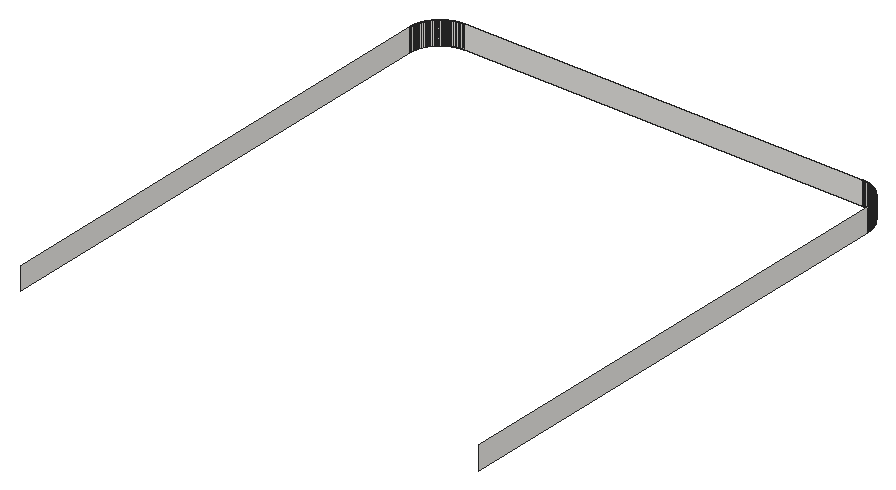
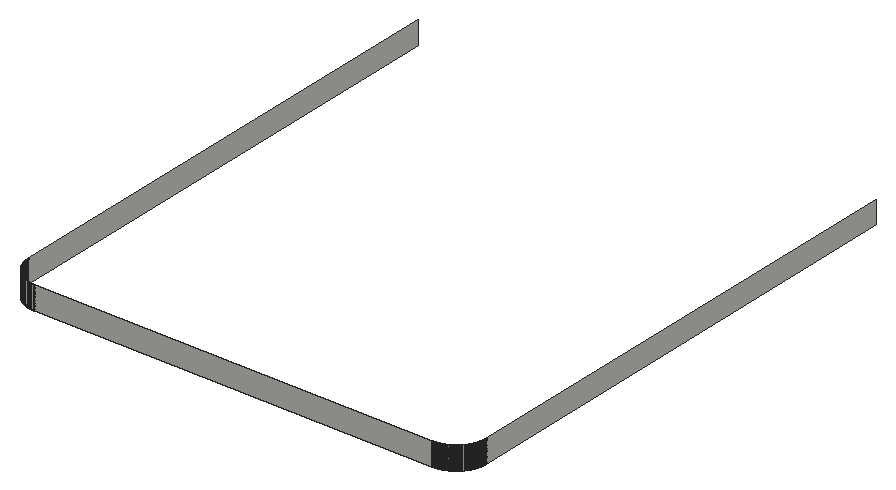
# SketchUp Ruby script. Lengths in inches.
U = 1.inch
M = Sketchup.active_model
def pt(a) = Geom::Point3d.new(a.map { |v| v * U })
def face(e, loops, mat)
  f = e.add_face(loops[0].map { |a| pt(a) })
  loops[1..].each { |l| e.add_face(l.map { |a| pt(a) }).erase! }
  f.material = f.back_material = mat if mat
  f
end
# faces: each face lists its corners as indices into pts; further lists are holes
def faces(e, pts, list, mat = nil) = list.each { |f| face(e, (f[0].is_a?(Array) ? f : [f]).map { |l| l.map { |i| pts[i] } }, mat) }
# xy, xz, yz: faces in a plane at the given z, y or x. An outline is a flat list of corners, or four numbers for a rectangle; further outlines are holes
def ring(l) = l.size == 4 ? [[l[0], l[1]], [l[2], l[1]], [l[2], l[3]], [l[0], l[3]]] : l.each_slice(2).to_a
def flat(e, list, mat, &to3) = list.each { |f| face(e, (f[0].is_a?(Array) ? f : [f]).map { |l| ring(l).map { |u, v| to3.(u, v) } }, mat) }
def xy(e, z, list, mat = nil) = flat(e, list, mat) { |x, y| [x, y, z] }
def xz(e, y, list, mat = nil) = flat(e, list, mat) { |x, z| [x, y, z] }
def yz(e, x, list, mat = nil) = flat(e, list, mat) { |y, z| [x, y, z] }
def lines(e, pts, list) = list.each { |a, b| e.add_line(pt(pts[a]), pt(pts[b])) }
# prism: a flat outline (further loops are holes) pulled along v
def prism(e, loops, v, mat = nil)
  f = face(e, loops, mat); d = Geom::Vector3d.new(v.map { |x| x * U })
  f.pushpull(f.normal.samedirection?(d) ? d.length : -d.length)
end
def box(e, o, s, mat = nil) = prism(e, [[o, [o[0] + s[0], o[1], o[2]], [o[0] + s[0], o[1] + s[1], o[2]], [o[0], o[1] + s[1], o[2]]]], [0, 0, s[2]], mat)
def at(x, y, z, deg = 0) = Geom::Transformation.translation(pt([x, y, z])) * Geom::Transformation.rotation(ORIGIN, Z_AXIS, deg.degrees)
def axes(o, x, y, z) = Geom::Transformation.new([*x, 0, *y, 0, *z, 0, *pt(o).to_a, 1])
def part(name) = M.definitions.add(name)
# library, detail: a bought-in or finely detailed component or shape, given as its bounding box
def library(name, o, s) = part(name).tap { |d| box(d.entities, o, s) }
def detail(e, o, s) = box(e.add_group.entities, o, s)
def put(e, d, t, mat = nil) = e.add_instance(d, t).tap { |i| i.material = mat if mat }
def group(e, t, mat = nil) = e.add_group.tap { |g| g.transformation = t; g.material = mat if mat }.entities
root = M.entities
M.materials.add("[Formica Graystone]").color = [224, 223, 219]
xz(root,444,[[17.6875,383.82,17.84,392.82],[17.84,383.82,18,392.82],[18,383.82,174,392.82],[174,383.82,174.16,392.82],[174.16,383.82,174.3125,392.82]],"[Formica Graystone]")
yz(root,6,[[241,383.82,432,392.82],[432,383.82,432.16,392.82],[432.16,383.82,432.3125,392.82]],"[Formica Graystone]")
yz(root,186,[[241,383.82,432,392.82],[432,383.82,432.16,392.82],[432.16,383.82,432.3125,392.82]],"[Formica Graystone]")
p = [[6.01,432.47,383.82],[6,432.3125,383.82],[6,432.3125,392.82],[6.01,432.47,392.82],[186,432.3125,383.82],[185.99,432.47,383.82],
  [185.99,432.47,392.82],[186,432.3125,392.82],[6.02,432.63,383.82],[6.02,432.63,392.82],[185.98,432.63,383.82],[185.98,432.63,392.82],
  [6.03,432.78,383.82],[6.03,432.78,392.82],[185.97,432.78,383.82],[185.97,432.78,392.82],[6.04,432.94,383.82],[6.04,432.94,392.82],
  [185.96,432.94,383.82],[185.96,432.94,392.82],[6.05,433.1,383.82],[6.05,433.1,392.82],[185.95,433.1,383.82],[185.95,433.1,392.82],
  [6.07,433.25,383.82],[6.07,433.25,392.82],[185.93,433.25,383.82],[185.93,433.25,392.82],[6.08,433.41,383.82],[6.08,433.41,392.82],
  [185.92,433.41,383.82],[185.92,433.41,392.82],[6.1,433.57,383.82],[6.1,433.57,392.82],[185.9,433.57,383.82],[185.9,433.57,392.82],
  [6.125,433.72,383.82],[6.125,433.72,392.82],[185.875,433.72,383.82],[185.875,433.72,392.82],[6.15,433.88,383.82],[6.15,433.88,392.82],
  [185.85,433.88,383.82],[185.85,433.88,392.82],[6.17,434.03,383.82],[6.17,434.03,392.82],[185.83,434.03,383.82],[185.83,434.03,392.82],
  [6.2,434.1875,383.82],[6.2,434.1875,392.82],[185.8,434.1875,383.82],[185.8,434.1875,392.82],[6.23,434.34,383.82],[6.23,434.34,392.82],
  [185.77,434.34,383.82],[185.77,434.34,392.82],[6.26,434.49,383.82],[6.26,434.49,392.82],[185.74,434.49,383.82],[185.74,434.49,392.82],
  [6.3,434.65,383.82],[6.3,434.65,392.82],[185.7,434.65,383.82],[185.7,434.65,392.82],[6.33,434.8,383.82],[6.33,434.8,392.82],
  [185.67,434.8,383.82],[185.67,434.8,392.82],[6.37,434.95,383.82],[6.37,434.95,392.82],[185.63,434.95,383.82],[185.63,434.95,392.82],
  [6.41,435.11,383.82],[6.41,435.11,392.82],[185.59,435.11,383.82],[185.59,435.11,392.82],[6.45,435.26,383.82],[6.45,435.26,392.82],
  [185.55,435.26,383.82],[185.55,435.26,392.82],[6.49,435.41,383.82],[6.49,435.41,392.82],[185.51,435.41,383.82],[185.51,435.41,392.82],
  [6.54,435.56,383.82],[6.54,435.56,392.82],[185.46,435.56,383.82],[185.46,435.56,392.82],[6.59,435.71,383.82],[6.59,435.71,392.82],
  [185.41,435.71,383.82],[185.41,435.71,392.82],[6.64,435.86,383.82],[6.64,435.86,392.82],[185.36,435.86,383.82],[185.36,435.86,392.82],
  [6.6875,436.01,383.82],[6.6875,436.01,392.82],[185.3125,436.01,383.82],[185.3125,436.01,392.82],[6.74,436.15,383.82],[6.74,436.15,392.82],
  [185.26,436.15,383.82],[185.26,436.15,392.82],[6.8,436.3,383.82],[6.8,436.3,392.82],[185.2,436.3,383.82],[185.2,436.3,392.82],
  [6.85,436.45,383.82],[6.85,436.45,392.82],[185.15,436.45,383.82],[185.15,436.45,392.82],[6.91,436.59,383.82],[6.91,436.59,392.82],
  [185.09,436.59,383.82],[185.09,436.59,392.82],[6.97,436.74,383.82],[6.97,436.74,392.82],[185.03,436.74,383.82],[185.03,436.74,392.82],
  [7.04,436.88,383.82],[7.04,436.88,392.82],[184.96,436.88,383.82],[184.96,436.88,392.82],[7.1,437.02,383.82],[7.1,437.02,392.82],
  [184.9,437.02,383.82],[184.9,437.02,392.82],[7.17,437.17,383.82],[7.17,437.17,392.82],[184.83,437.17,383.82],[184.83,437.17,392.82],
  [7.24,437.31,383.82],[7.24,437.31,392.82],[184.76,437.31,383.82],[184.76,437.31,392.82],[7.31,437.45,383.82],[7.31,437.45,392.82],
  [184.69,437.45,383.82],[184.69,437.45,392.82],[7.38,437.59,383.82],[7.38,437.59,392.82],[184.62,437.59,383.82],[184.62,437.59,392.82],
  [7.45,437.73,383.82],[7.45,437.73,392.82],[184.55,437.73,383.82],[184.55,437.73,392.82],[7.53,437.86,383.82],[7.53,437.86,392.82],
  [184.47,437.86,383.82],[184.47,437.86,392.82],[7.61,438,383.82],[7.61,438,392.82],[184.39,438,383.82],[184.39,438,392.82],
  [7.6875,438.14,383.82],[7.6875,438.14,392.82],[184.3125,438.14,383.82],[184.3125,438.14,392.82],[7.77,438.27,383.82],[7.77,438.27,392.82],
  [184.23,438.27,383.82],[184.23,438.27,392.82],[7.85,438.4,383.82],[7.85,438.4,392.82],[184.15,438.4,383.82],[184.15,438.4,392.82],
  [7.9375,438.54,383.82],[7.9375,438.54,392.82],[184.0625,438.54,383.82],[184.0625,438.54,392.82],[8.02,438.67,383.82],[8.02,438.67,392.82],
  [183.98,438.67,383.82],[183.98,438.67,392.82],[8.11,438.8,383.82],[8.11,438.8,392.82],[183.89,438.8,383.82],[183.89,438.8,392.82],
  [8.2,438.93,383.82],[8.2,438.93,392.82],[183.8,438.93,383.82],[183.8,438.93,392.82],[8.29,439.05,383.82],[8.29,439.05,392.82],
  [183.71,439.05,383.82],[183.71,439.05,392.82],[8.38,439.18,383.82],[8.38,439.18,392.82],[183.62,439.18,383.82],[183.62,439.18,392.82],
  [8.48,439.31,383.82],[8.48,439.31,392.82],[183.52,439.31,383.82],[183.52,439.31,392.82],[8.58,439.43,383.82],[8.58,439.43,392.82],
  [183.42,439.43,383.82],[183.42,439.43,392.82],[8.67,439.55,383.82],[8.67,439.55,392.82],[183.33,439.55,383.82],[183.33,439.55,392.82],
  [8.77,439.67,383.82],[8.77,439.67,392.82],[183.23,439.67,383.82],[183.23,439.67,392.82],[8.875,439.79,383.82],[8.875,439.79,392.82],
  [183.125,439.79,383.82],[183.125,439.79,392.82],[8.98,439.91,383.82],[8.98,439.91,392.82],[183.02,439.91,383.82],[183.02,439.91,392.82],
  [9.08,440.03,383.82],[9.08,440.03,392.82],[182.92,440.03,383.82],[182.92,440.03,392.82],[9.1875,440.15,383.82],[9.1875,440.15,392.82],
  [182.8125,440.15,383.82],[182.8125,440.15,392.82],[9.3,440.26,383.82],[9.3,440.26,392.82],[182.7,440.26,383.82],[182.7,440.26,392.82],
  [9.4,440.375,383.82],[9.4,440.375,392.82],[182.6,440.375,383.82],[182.6,440.375,392.82],[9.51,440.49,383.82],[9.51,440.49,392.82],
  [182.49,440.49,383.82],[182.49,440.49,392.82],[9.625,440.6,383.82],[9.625,440.6,392.82],[182.375,440.6,383.82],[182.375,440.6,392.82],
  [9.74,440.7,383.82],[9.74,440.7,392.82],[182.26,440.7,383.82],[182.26,440.7,392.82],[9.85,440.8125,383.82],[9.85,440.8125,392.82],
  [182.15,440.8125,383.82],[182.15,440.8125,392.82],[9.97,440.92,383.82],[9.97,440.92,392.82],[182.03,440.92,383.82],[182.03,440.92,392.82],
  [10.09,441.02,383.82],[10.09,441.02,392.82],[181.91,441.02,383.82],[181.91,441.02,392.82],[10.21,441.125,383.82],[10.21,441.125,392.82],
  [181.79,441.125,383.82],[181.79,441.125,392.82],[10.33,441.23,383.82],[10.33,441.23,392.82],[181.67,441.23,383.82],[181.67,441.23,392.82],
  [10.45,441.33,383.82],[10.45,441.33,392.82],[181.55,441.33,383.82],[181.55,441.33,392.82],[10.57,441.42,383.82],[10.57,441.42,392.82],
  [181.43,441.42,383.82],[181.43,441.42,392.82],[10.69,441.52,383.82],[10.69,441.52,392.82],[181.31,441.52,383.82],[181.31,441.52,392.82],
  [10.82,441.62,383.82],[10.82,441.62,392.82],[181.18,441.62,383.82],[181.18,441.62,392.82],[10.95,441.71,383.82],[10.95,441.71,392.82],
  [181.05,441.71,383.82],[181.05,441.71,392.82],[11.07,441.8,383.82],[11.07,441.8,392.82],[180.93,441.8,383.82],[180.93,441.8,392.82],
  [11.2,441.89,383.82],[11.2,441.89,392.82],[180.8,441.89,383.82],[180.8,441.89,392.82],[11.33,441.98,383.82],[11.33,441.98,392.82],
  [180.67,441.98,383.82],[180.67,441.98,392.82],[11.46,442.0625,383.82],[11.46,442.0625,392.82],[180.54,442.0625,383.82],[180.54,442.0625,392.82],
  [11.6,442.15,383.82],[11.6,442.15,392.82],[11.73,442.23,383.82],[11.73,442.23,392.82],[180.4,442.15,383.82],[180.27,442.23,383.82],
  [180.27,442.23,392.82],[180.4,442.15,392.82],[11.86,442.3125,383.82],[11.86,442.3125,392.82],[180.14,442.3125,383.82],[180.14,442.3125,392.82],
  [12,442.39,383.82],[12,442.39,392.82],[180,442.39,383.82],[180,442.39,392.82],[12.14,442.47,383.82],[12.14,442.47,392.82],
  [179.86,442.47,383.82],[179.86,442.47,392.82],[12.27,442.55,383.82],[12.27,442.55,392.82],[12.41,442.62,383.82],[12.41,442.62,392.82],
  [179.73,442.55,383.82],[179.59,442.62,383.82],[179.59,442.62,392.82],[179.73,442.55,392.82],[12.55,442.69,383.82],[12.55,442.69,392.82],
  [179.45,442.69,383.82],[179.45,442.69,392.82],[12.69,442.76,383.82],[12.69,442.76,392.82],[179.31,442.76,383.82],[179.31,442.76,392.82],
  [12.83,442.83,383.82],[12.83,442.83,392.82],[12.98,442.9,383.82],[12.98,442.9,392.82],[179.17,442.83,383.82],[179.02,442.9,383.82],
  [179.02,442.9,392.82],[179.17,442.83,392.82],[13.12,442.96,383.82],[13.12,442.96,392.82],[178.88,442.96,383.82],[178.88,442.96,392.82],
  [13.26,443.03,383.82],[13.26,443.03,392.82],[13.41,443.09,383.82],[13.41,443.09,392.82],[178.74,443.03,383.82],[178.59,443.09,383.82],
  [178.59,443.09,392.82],[178.74,443.03,392.82],[13.55,443.15,383.82],[13.55,443.15,392.82],[13.7,443.2,383.82],[13.7,443.2,392.82],
  [178.45,443.15,383.82],[178.3,443.2,383.82],[178.3,443.2,392.82],[178.45,443.15,392.82],[13.85,443.26,383.82],[13.85,443.26,392.82],
  [178.15,443.26,383.82],[178.15,443.26,392.82],[13.99,443.3125,383.82],[13.99,443.3125,392.82],[14.14,443.36,383.82],[14.14,443.36,392.82],
  [178.01,443.3125,383.82],[177.86,443.36,383.82],[177.86,443.36,392.82],[178.01,443.3125,392.82],[14.29,443.41,383.82],[14.29,443.41,392.82],
  [14.44,443.46,383.82],[14.44,443.46,392.82],[177.71,443.41,383.82],[177.56,443.46,383.82],[177.56,443.46,392.82],[177.71,443.41,392.82],
  [14.59,443.51,383.82],[14.59,443.51,392.82],[14.74,443.55,383.82],[14.74,443.55,392.82],[14.89,443.59,383.82],[14.89,443.59,392.82],
  [177.26,443.55,383.82],[177.11,443.59,383.82],[177.11,443.59,392.82],[177.26,443.55,392.82],[177.41,443.51,383.82],[177.41,443.51,392.82],
  [15.05,443.63,383.82],[15.05,443.63,392.82],[15.2,443.67,383.82],[15.2,443.67,392.82],[176.95,443.63,383.82],[176.8,443.67,383.82],
  [176.8,443.67,392.82],[176.95,443.63,392.82],[15.35,443.7,383.82],[15.35,443.7,392.82],[15.51,443.74,383.82],[15.51,443.74,392.82],
  [15.66,443.77,383.82],[15.66,443.77,392.82],[176.49,443.74,383.82],[176.34,443.77,383.82],[176.34,443.77,392.82],[176.49,443.74,392.82],
  [176.65,443.7,383.82],[176.65,443.7,392.82],[15.8125,443.8,383.82],[15.8125,443.8,392.82],[15.97,443.83,383.82],[15.97,443.83,392.82],
  [16.12,443.85,383.82],[16.12,443.85,392.82],[176.03,443.83,383.82],[175.88,443.85,383.82],[175.88,443.85,392.82],[176.03,443.83,392.82],
  [176.1875,443.8,383.82],[176.1875,443.8,392.82],[16.28,443.875,383.82],[16.28,443.875,392.82],[16.43,443.9,383.82],[16.43,443.9,392.82],
  [16.59,443.92,383.82],[16.59,443.92,392.82],[16.75,443.93,383.82],[16.75,443.93,392.82],[16.9,443.95,383.82],[16.9,443.95,392.82],
  [17.06,443.96,383.82],[17.06,443.96,392.82],[175.1,443.95,383.82],[174.94,443.96,383.82],[174.94,443.96,392.82],[175.1,443.95,392.82],
  [175.25,443.93,383.82],[175.25,443.93,392.82],[175.41,443.92,383.82],[175.41,443.92,392.82],[175.57,443.9,383.82],[175.57,443.9,392.82],
  [175.72,443.875,383.82],[175.72,443.875,392.82],[17.22,443.97,383.82],[17.22,443.97,392.82],[17.37,443.98,383.82],[17.37,443.98,392.82],
  [17.53,443.99,383.82],[17.53,443.99,392.82],[17.6875,444,383.82],[17.6875,444,392.82],[174.47,443.99,383.82],[174.3125,444,383.82],
  [174.3125,444,392.82],[174.47,443.99,392.82],[174.63,443.98,383.82],[174.63,443.98,392.82],[174.78,443.97,383.82],[174.78,443.97,392.82]]
faces(root,p,[[0,1,2,3],[4,5,6,7],[8,0,3,9],[5,10,11,6],[12,8,9,13],[10,14,15,11],[16,12,13,17],[14,18,19,15],
  [20,16,17,21],[18,22,23,19],[24,20,21,25],[22,26,27,23],[28,24,25,29],[26,30,31,27],[32,28,29,33],[30,34,35,31],
  [36,32,33,37],[34,38,39,35],[40,36,37,41],[38,42,43,39],[44,40,41,45],[42,46,47,43],[48,44,45,49],[46,50,51,47],
  [52,48,49,53],[50,54,55,51],[56,52,53,57],[54,58,59,55],[60,56,57,61],[58,62,63,59],[64,60,61,65],[62,66,67,63],
  [68,64,65,69],[66,70,71,67],[72,68,69,73],[70,74,75,71],[76,72,73,77],[74,78,79,75],[80,76,77,81],[78,82,83,79],
  [84,80,81,85],[82,86,87,83],[88,84,85,89],[86,90,91,87],[92,88,89,93],[90,94,95,91],[96,92,93,97],[94,98,99,95],
  [100,96,97,101],[98,102,103,99],[104,100,101,105],[102,106,107,103],[108,104,105,109],[106,110,111,107],[112,108,109,113],[110,114,115,111],
  [116,112,113,117],[114,118,119,115],[120,116,117,121],[118,122,123,119],[124,120,121,125],[122,126,127,123],[128,124,125,129],[126,130,131,127],
  [132,128,129,133],[130,134,135,131],[136,132,133,137],[134,138,139,135],[140,136,137,141],[138,142,143,139],[144,140,141,145],[142,146,147,143],
  [148,144,145,149],[146,150,151,147],[152,148,149,153],[150,154,155,151],[156,152,153,157],[154,158,159,155],[160,156,157,161],[158,162,163,159],
  [164,160,161,165],[162,166,167,163],[168,164,165,169],[166,170,171,167],[172,168,169,173],[170,174,175,171],[176,172,173,177],[174,178,179,175],
  [180,176,177,181],[178,182,183,179],[184,180,181,185],[182,186,187,183],[188,184,185,189],[186,190,191,187],[192,188,189,193],[190,194,195,191],
  [196,192,193,197],[194,198,199,195],[200,196,197,201],[198,202,203,199],[204,200,201,205],[202,206,207,203],[208,204,205,209],[206,210,211,207],
  [212,208,209,213],[210,214,215,211],[216,212,213,217],[214,218,219,215],[220,216,217,221],[218,222,223,219],[224,220,221,225],[222,226,227,223],
  [228,224,225,229],[226,230,231,227],[232,228,229,233],[230,234,235,231],[236,232,233,237],[234,238,239,235],[240,236,237,241],[238,242,243,239],
  [244,240,241,245],[242,246,247,243],[248,244,245,249],[246,250,251,247],[252,248,249,253],[250,254,255,251],[256,252,253,257],[254,258,259,255],
  [260,256,257,261],[258,262,263,259],[264,260,261,265],[262,266,267,263],[268,264,265,269],[266,270,271,267],[272,268,269,273],[270,274,275,271],
  [276,272,273,277],[274,278,279,275],[280,276,277,281],[278,282,283,279],[284,280,281,285],[282,286,287,283],[288,284,285,289],[286,290,291,287],
  [292,288,289,293],[290,294,295,291],[296,292,293,297],[294,298,299,295],[300,296,297,301],[302,300,301,303],[304,305,306,307],[298,304,307,299],
  [308,302,303,309],[305,310,311,306],[312,308,309,313],[310,314,315,311],[316,312,313,317],[314,318,319,315],[320,316,317,321],[322,320,321,323],
  [324,325,326,327],[318,324,327,319],[328,322,323,329],[325,330,331,326],[332,328,329,333],[330,334,335,331],[336,332,333,337],[338,336,337,339],
  [340,341,342,343],[334,340,343,335],[344,338,339,345],[341,346,347,342],[348,344,345,349],[350,348,349,351],[352,353,354,355],[346,352,355,347],
  [356,350,351,357],[358,356,357,359],[360,361,362,363],[353,360,363,354],[364,358,359,365],[361,366,367,362],[368,364,365,369],[370,368,369,371],
  [372,373,374,375],[366,372,375,367],[376,370,371,377],[378,376,377,379],[380,381,382,383],[373,380,383,374],[384,378,379,385],[386,384,385,387],
  [388,386,387,389],[390,391,392,393],[394,390,393,395],[381,394,395,382],[396,388,389,397],[398,396,397,399],[400,401,402,403],[391,400,403,392],
  [404,398,399,405],[406,404,405,407],[408,406,407,409],[410,411,412,413],[414,410,413,415],[401,414,415,402],[416,408,409,417],[418,416,417,419],
  [420,418,419,421],[422,423,424,425],[426,422,425,427],[411,426,427,412],[428,420,421,429],[430,428,429,431],[432,430,431,433],[434,432,433,435],
  [436,434,435,437],[438,436,437,439],[440,441,442,443],[444,440,443,445],[446,444,445,447],[448,446,447,449],[450,448,449,451],[423,450,451,424],
  [452,438,439,453],[454,452,453,455],[456,454,455,457],[458,456,457,459],[460,461,462,463],[464,460,463,465],[466,464,465,467],[441,466,467,442]],"[Formica Graystone]")
